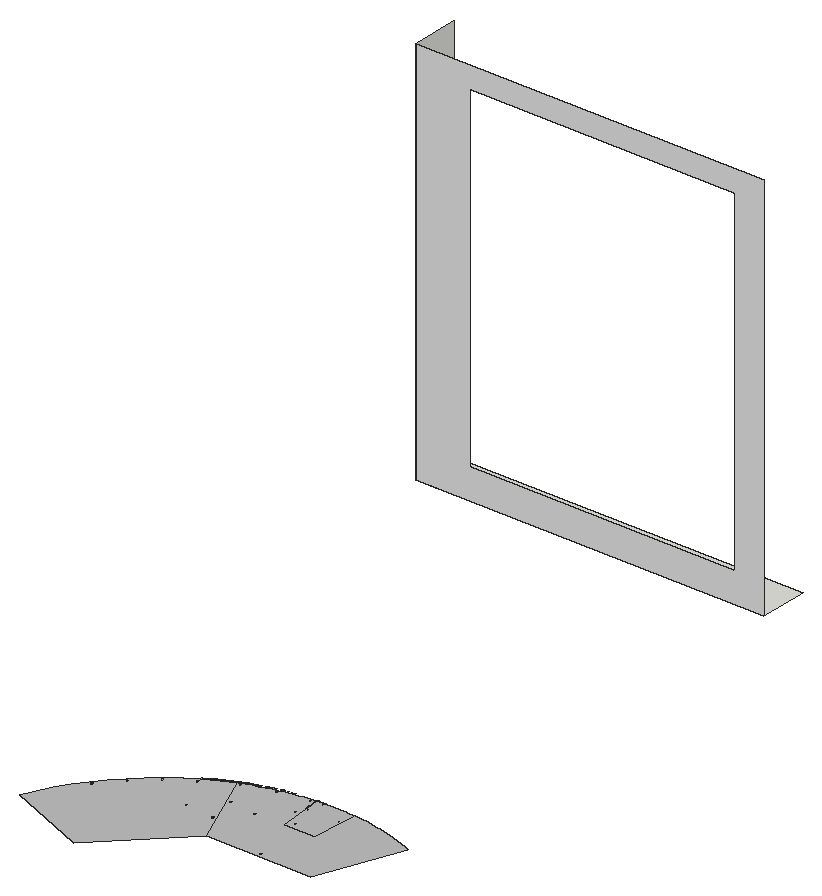
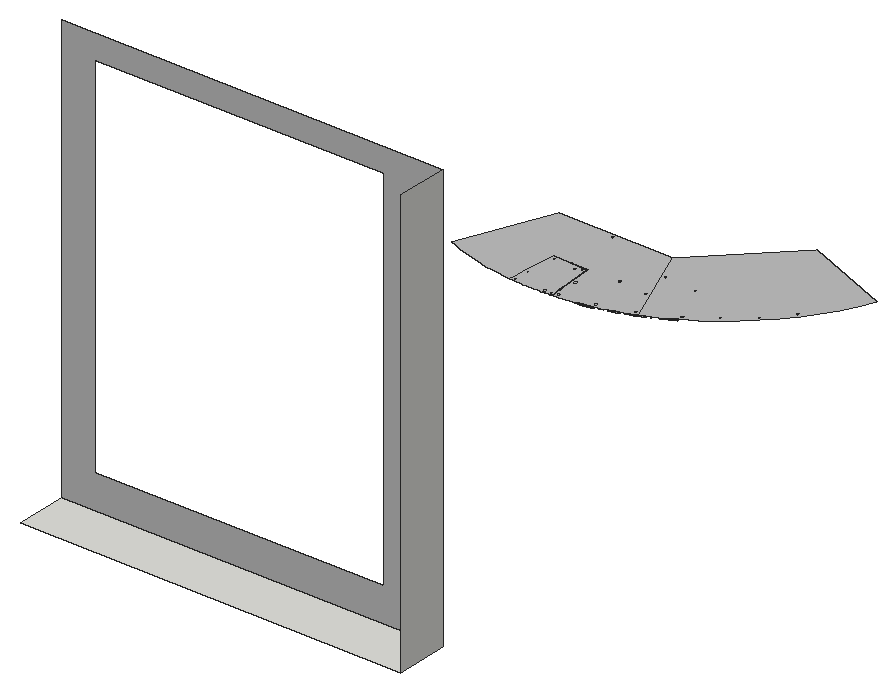
# SketchUp Ruby script. Lengths in inches.
U = 1.inch
M = Sketchup.active_model
def pt(a) = Geom::Point3d.new(a.map { |v| v * U })
def face(e, loops, mat)
  f = e.add_face(loops[0].map { |a| pt(a) })
  loops[1..].each { |l| e.add_face(l.map { |a| pt(a) }).erase! }
  f.material = f.back_material = mat if mat
  f
end
# faces: each face lists its corners as indices into pts; further lists are holes
def faces(e, pts, list, mat = nil) = list.each { |f| face(e, (f[0].is_a?(Array) ? f : [f]).map { |l| l.map { |i| pts[i] } }, mat) }
# xy, xz, yz: faces in a plane at the given z, y or x. An outline is a flat list of corners, or four numbers for a rectangle; further outlines are holes
def ring(l) = l.size == 4 ? [[l[0], l[1]], [l[2], l[1]], [l[2], l[3]], [l[0], l[3]]] : l.each_slice(2).to_a
def flat(e, list, mat, &to3) = list.each { |f| face(e, (f[0].is_a?(Array) ? f : [f]).map { |l| ring(l).map { |u, v| to3.(u, v) } }, mat) }
def xy(e, z, list, mat = nil) = flat(e, list, mat) { |x, y| [x, y, z] }
def xz(e, y, list, mat = nil) = flat(e, list, mat) { |x, z| [x, y, z] }
def yz(e, x, list, mat = nil) = flat(e, list, mat) { |y, z| [x, y, z] }
def lines(e, pts, list) = list.each { |a, b| e.add_line(pt(pts[a]), pt(pts[b])) }
# prism: a flat outline (further loops are holes) pulled along v
def prism(e, loops, v, mat = nil)
  f = face(e, loops, mat); d = Geom::Vector3d.new(v.map { |x| x * U })
  f.pushpull(f.normal.samedirection?(d) ? d.length : -d.length)
end
def box(e, o, s, mat = nil) = prism(e, [[o, [o[0] + s[0], o[1], o[2]], [o[0] + s[0], o[1] + s[1], o[2]], [o[0], o[1] + s[1], o[2]]]], [0, 0, s[2]], mat)
def at(x, y, z, deg = 0) = Geom::Transformation.translation(pt([x, y, z])) * Geom::Transformation.rotation(ORIGIN, Z_AXIS, deg.degrees)
def axes(o, x, y, z) = Geom::Transformation.new([*x, 0, *y, 0, *z, 0, *pt(o).to_a, 1])
def part(name) = M.definitions.add(name)
# library, detail: a bought-in or finely detailed component or shape, given as its bounding box
def library(name, o, s) = part(name).tap { |d| box(d.entities, o, s) }
def detail(e, o, s) = box(e.add_group.entities, o, s)
def put(e, d, t, mat = nil) = e.add_instance(d, t).tap { |i| i.material = mat if mat }
def group(e, t, mat = nil) = e.add_group.tap { |g| g.transformation = t; g.material = mat if mat }.entities
root = M.entities
M.materials.add("[Metal_Steel_Textured_White]").color = [191, 191, 191]
M.materials.add("[Polished Concrete Old]").color = [229, 229, 229]
xy(root,3.625,[[116.615,243.402,158.149,249.09]])
xy(root,3.625,[[[134.847,169.578,125.229,173.5625,125.948,175.149,126.769,176.685,127.689,178.164,128.703,179.579,129.808,180.926,130.999,182.197,132.27,183.387,133.616,184.492,135.032,185.507,136.511,186.426,138.047,187.247,139.633,187.966,143.617,178.348],[141.048,176.255,141.071,176.258,141.092,176.267,141.111,176.281,141.125,176.299,141.134,176.321,141.137,176.344,141.134,176.367,141.125,176.388,141.111,176.407,141.092,176.421,141.071,176.43,141.048,176.433,141.025,176.43,141.003,176.421,140.985,176.407,140.971,176.388,140.962,176.367,140.959,176.344,140.962,176.321,140.971,176.299,140.985,176.281,141.003,176.267,141.025,176.258],[138.462,181.667,138.485,181.67,138.507,181.679,138.525,181.693,138.539,181.712,138.548,181.733,138.551,181.756,138.548,181.779,138.539,181.801,138.525,181.819,138.507,181.833,138.485,181.842,138.462,181.845,138.439,181.842,138.418,181.833,138.399,181.819,138.385,181.801,138.376,181.779,138.373,181.756,138.376,181.733,138.385,181.712,138.399,181.693,138.418,181.679,138.439,181.67],[125.754,173.688,125.777,173.691,125.798,173.7,125.817,173.714,125.831,173.733,125.84,173.754,125.843,173.777,125.84,173.8,125.831,173.822,125.817,173.84,125.798,173.854,125.777,173.863,125.754,173.866,125.731,173.863,125.709,173.854,125.691,173.84,125.677,173.822,125.668,173.8,125.665,173.777,125.668,173.754,125.677,173.733,125.691,173.714,125.709,173.7,125.731,173.691],[128.754,172.446,128.777,172.449,128.798,172.458,128.816,172.472,128.831,172.49,128.839,172.512,128.843,172.535,128.839,172.558,128.831,172.579,128.816,172.597,128.798,172.612,128.777,172.62,128.754,172.624,128.731,172.62,128.709,172.612,128.691,172.597,128.677,172.579,128.668,172.558,128.665,172.535,128.668,172.512,128.677,172.49,128.691,172.472,128.709,172.458,128.731,172.449],[143.146,178.353,143.169,178.356,143.19,178.365,143.209,178.379,143.223,178.397,143.232,178.419,143.235,178.442,143.232,178.465,143.223,178.486,143.209,178.505,143.19,178.519,143.169,178.528,143.146,178.531,143.123,178.528,143.101,178.519,143.083,178.505,143.069,178.486,143.06,178.465,143.057,178.442,143.06,178.419,143.069,178.397,143.083,178.379,143.101,178.365,143.123,178.356],[134.754,169.961,134.777,169.964,134.798,169.972,134.816,169.987,134.831,170.005,134.839,170.026,134.842,170.049,134.839,170.072,134.831,170.094,134.816,170.112,134.798,170.126,134.777,170.135,134.754,170.138,134.731,170.135,134.709,170.126,134.691,170.112,134.677,170.094,134.668,170.072,134.665,170.049,134.668,170.026,134.677,170.005,134.691,169.987,134.709,169.972,134.731,169.964],[140.661,184.353,140.684,184.356,140.705,184.365,140.724,184.379,140.738,184.397,140.747,184.419,140.75,184.442,140.747,184.465,140.738,184.486,140.724,184.505,140.705,184.519,140.684,184.528,140.661,184.531,140.638,184.528,140.616,184.519,140.598,184.505,140.584,184.486,140.575,184.465,140.572,184.442,140.575,184.419,140.584,184.397,140.598,184.379,140.616,184.365,140.638,184.356],[136.48,185.857,136.503,185.86,136.525,185.869,136.543,185.883,136.557,185.902,136.566,185.923,136.569,185.946,136.566,185.969,136.557,185.991,136.543,186.009,136.525,186.023,136.503,186.032,136.48,186.035,136.457,186.032,136.436,186.023,136.418,186.009,136.403,185.991,136.395,185.969,136.392,185.946,136.395,185.923,136.403,185.902,136.418,185.883,136.436,185.869,136.457,185.86],[131.754,171.203,131.777,171.206,131.798,171.215,131.816,171.229,131.831,171.248,131.839,171.269,131.842,171.292,131.839,171.315,131.831,171.336,131.816,171.355,131.798,171.369,131.777,171.378,131.754,171.381,131.731,171.378,131.709,171.369,131.691,171.355,131.677,171.336,131.668,171.315,131.665,171.292,131.668,171.269,131.677,171.248,131.691,171.229,131.709,171.215,131.731,171.206],[131.439,174.644,131.462,174.647,131.483,174.656,131.502,174.67,131.516,174.689,131.525,174.71,131.528,174.733,131.525,174.756,131.516,174.778,131.502,174.796,131.483,174.81,131.462,174.819,131.439,174.822,131.416,174.819,131.395,174.81,131.376,174.796,131.362,174.778,131.353,174.756,131.35,174.733,131.353,174.71,131.362,174.689,131.376,174.67,131.395,174.656,131.416,174.647],[138.95,174.157,138.973,174.16,138.994,174.169,139.013,174.183,139.027,174.201,139.036,174.223,139.039,174.246,139.036,174.269,139.027,174.29,139.013,174.308,138.994,174.323,138.973,174.331,138.95,174.334,138.927,174.331,138.905,174.323,138.887,174.308,138.873,174.29,138.864,174.269,138.861,174.246,138.864,174.223,138.873,174.201,138.887,174.183,138.905,174.169,138.927,174.16],[127.249,176.626,127.272,176.629,127.293,176.638,127.312,176.652,127.326,176.67,127.335,176.692,127.338,176.715,127.335,176.738,127.326,176.759,127.312,176.778,127.293,176.792,127.272,176.801,127.249,176.804,127.226,176.801,127.205,176.792,127.186,176.778,127.172,176.759,127.163,176.738,127.16,176.715,127.163,176.692,127.172,176.67,127.186,176.652,127.205,176.638,127.226,176.629],[133.754,184.005,133.777,184.008,133.798,184.017,133.816,184.031,133.831,184.05,133.839,184.071,133.843,184.094,133.839,184.117,133.831,184.139,133.816,184.157,133.798,184.171,133.777,184.18,133.754,184.183,133.731,184.18,133.709,184.171,133.691,184.157,133.677,184.139,133.668,184.117,133.665,184.094,133.668,184.071,133.677,184.05,133.691,184.031,133.709,184.017,133.731,184.008],[129.101,179.353,129.124,179.356,129.146,179.365,129.164,179.379,129.178,179.397,129.187,179.419,129.19,179.442,129.187,179.465,129.178,179.486,129.164,179.505,129.146,179.519,129.124,179.528,129.101,179.531,129.078,179.528,129.057,179.519,129.038,179.505,129.024,179.486,129.015,179.465,129.012,179.442,129.015,179.419,129.024,179.397,129.038,179.379,129.057,179.365,129.078,179.356],[133.78,176.985,133.803,176.988,133.825,176.997,133.843,177.011,133.857,177.03,133.866,177.051,133.869,177.074,133.866,177.097,133.857,177.119,133.843,177.137,133.825,177.151,133.803,177.16,133.78,177.163,133.757,177.16,133.736,177.151,133.717,177.137,133.703,177.119,133.694,177.097,133.691,177.074,133.694,177.051,133.703,177.03,133.717,177.011,133.736,176.997,133.757,176.988],[136.852,172.059,136.875,172.062,136.896,172.071,136.914,172.085,136.929,172.103,136.9375,172.124,136.941,172.147,136.9375,172.17,136.929,172.192,136.914,172.21,136.896,172.224,136.875,172.233,136.852,172.236,136.829,172.233,136.807,172.224,136.789,172.21,136.775,172.192,136.766,172.17,136.763,172.147,136.766,172.124,136.775,172.103,136.789,172.085,136.807,172.071,136.829,172.062],[131.281,181.826,131.304,181.829,131.325,181.837,131.344,181.852,131.358,181.87,131.367,181.891,131.37,181.914,131.367,181.9375,131.358,181.959,131.344,181.977,131.325,181.991,131.304,182,131.281,182.003,131.258,182,131.236,181.991,131.218,181.977,131.204,181.959,131.195,181.9375,131.192,181.914,131.195,181.891,131.204,181.87,131.218,181.852,131.236,181.837,131.258,181.829],[136.121,179.326,136.144,179.329,136.166,179.338,136.184,179.352,136.198,179.371,136.207,179.392,136.21,179.415,136.207,179.438,136.198,179.46,136.184,179.478,136.166,179.492,136.144,179.501,136.121,179.504,136.098,179.501,136.077,179.492,136.058,179.478,136.044,179.46,136.035,179.438,136.032,179.415,136.035,179.392,136.044,179.371,136.058,179.352,136.077,179.338,136.098,179.329],[139.418,187.353,139.441,187.356,139.462,187.365,139.481,187.379,139.495,187.397,139.504,187.419,139.507,187.442,139.504,187.465,139.495,187.486,139.481,187.505,139.462,187.519,139.441,187.528,139.418,187.531,139.395,187.528,139.374,187.519,139.355,187.505,139.341,187.486,139.332,187.465,139.329,187.442,139.332,187.419,139.341,187.397,139.355,187.379,139.374,187.365,139.395,187.356],[141.903,181.353,141.926,181.356,141.948,181.365,141.966,181.379,141.98,181.397,141.989,181.419,141.992,181.442,141.989,181.465,141.98,181.486,141.966,181.505,141.948,181.519,141.926,181.528,141.903,181.531,141.88,181.528,141.859,181.519,141.84,181.505,141.826,181.486,141.817,181.465,141.814,181.442,141.817,181.419,141.826,181.397,141.84,181.379,141.859,181.365,141.88,181.356]],[[143.617,178.348,139.633,187.966,140.262,188.217,140.897,188.452,141.538,188.671,142.185,188.874,142.836,189.06,143.492,189.229,144.152,189.382,144.816,189.518,145.483,189.636,146.152,189.738,146.824,189.823,147.498,189.891,147.513,189.727,147.542,189.396,147.548,189.326,147.59,188.846,147.62,188.494,147.627,188.414,147.634,188.34,147.643,188.234,147.655,188.101,147.97,184.503,151.666,184.503,151.981,188.101,151.993,188.234,152.002,188.34,152.094,189.396,152.123,189.727,152.138,189.891,152.812,189.823,153.484,189.738,154.153,189.636,154.82,189.518,155.484,189.382,156.144,189.229,156.8,189.06,157.451,188.874,158.097,188.671,158.738,188.452,159.374,188.217,160.003,187.966,156.019,178.348],[147.136,189.366,147.159,189.369,147.18,189.378,147.198,189.392,147.213,189.411,147.222,189.432,147.225,189.455,147.222,189.478,147.213,189.5,147.198,189.518,147.18,189.532,147.159,189.541,147.136,189.544,147.113,189.541,147.091,189.532,147.073,189.518,147.059,189.5,147.05,189.478,147.047,189.455,147.05,189.432,147.059,189.411,147.073,189.392,147.091,189.378,147.113,189.369],[152.5,189.366,152.523,189.369,152.545,189.378,152.563,189.392,152.577,189.411,152.586,189.432,152.589,189.455,152.586,189.478,152.577,189.5,152.563,189.518,152.545,189.532,152.523,189.541,152.5,189.544,152.477,189.541,152.456,189.532,152.437,189.518,152.423,189.5,152.414,189.478,152.411,189.455,152.414,189.432,152.423,189.411,152.437,189.392,152.456,189.378,152.477,189.369],[142.641,181.658,142.664,181.661,142.685,181.67,142.704,181.684,142.718,181.703,142.727,181.724,142.73,181.747,142.727,181.77,142.718,181.792,142.704,181.81,142.685,181.824,142.664,181.833,142.641,181.836,142.618,181.833,142.597,181.824,142.578,181.81,142.564,181.792,142.555,181.77,142.552,181.747,142.555,181.724,142.564,181.703,142.578,181.684,142.597,181.67,142.618,181.661],[159.48,187.658,159.503,187.661,159.525,187.67,159.543,187.684,159.557,187.703,159.566,187.724,159.569,187.747,159.566,187.77,159.557,187.792,159.543,187.81,159.525,187.824,159.503,187.833,159.48,187.836,159.457,187.833,159.436,187.824,159.417,187.81,159.403,187.792,159.394,187.77,159.391,187.747,159.394,187.724,159.403,187.703,159.417,187.684,159.436,187.67,159.457,187.661],[156.995,181.658,157.018,181.661,157.039,181.67,157.058,181.684,157.072,181.703,157.081,181.724,157.084,181.747,157.081,181.77,157.072,181.792,157.058,181.81,157.039,181.824,157.018,181.833,156.995,181.836,156.972,181.833,156.95,181.824,156.932,181.81,156.918,181.792,156.909,181.77,156.906,181.747,156.909,181.724,156.918,181.703,156.932,181.684,156.95,181.67,156.972,181.661],[141.398,184.658,141.421,184.661,141.443,184.67,141.461,184.684,141.475,184.703,141.484,184.724,141.487,184.747,141.484,184.77,141.475,184.792,141.461,184.81,141.443,184.824,141.421,184.833,141.398,184.836,141.375,184.833,141.354,184.824,141.335,184.81,141.321,184.792,141.3125,184.77,141.309,184.747,141.3125,184.724,141.321,184.703,141.335,184.684,141.354,184.67,141.375,184.661],[158.237,184.658,158.26,184.661,158.282,184.67,158.3,184.684,158.314,184.703,158.323,184.724,158.326,184.747,158.323,184.77,158.314,184.792,158.3,184.81,158.282,184.824,158.26,184.833,158.237,184.836,158.214,184.833,158.193,184.824,158.175,184.81,158.16,184.792,158.152,184.77,158.149,184.747,158.152,184.724,158.16,184.703,158.175,184.684,158.193,184.67,158.214,184.661],[140.156,187.658,140.179,187.661,140.2,187.67,140.219,187.684,140.233,187.703,140.242,187.724,140.245,187.747,140.242,187.77,140.233,187.792,140.219,187.81,140.2,187.824,140.179,187.833,140.156,187.836,140.133,187.833,140.111,187.824,140.093,187.81,140.079,187.792,140.07,187.77,140.067,187.747,140.07,187.724,140.079,187.703,140.093,187.684,140.111,187.67,140.133,187.661],[156.049,188.753,156.072,188.756,156.093,188.764,156.112,188.779,156.126,188.797,156.135,188.818,156.138,188.841,156.135,188.864,156.126,188.886,156.112,188.904,156.093,188.918,156.072,188.927,156.049,188.93,156.026,188.927,156.004,188.918,155.986,188.904,155.972,188.886,155.963,188.864,155.96,188.841,155.963,188.818,155.972,188.797,155.986,188.779,156.004,188.764,156.026,188.756],[143.884,178.658,143.907,178.661,143.928,178.67,143.946,178.684,143.961,178.703,143.969,178.724,143.972,178.747,143.969,178.77,143.961,178.792,143.946,178.81,143.928,178.824,143.907,178.833,143.884,178.836,143.861,178.833,143.839,178.824,143.821,178.81,143.807,178.792,143.798,178.77,143.795,178.747,143.798,178.724,143.807,178.703,143.821,178.684,143.839,178.67,143.861,178.661],[143.587,188.753,143.61,188.756,143.631,188.764,143.65,188.779,143.664,188.797,143.673,188.818,143.676,188.841,143.673,188.864,143.664,188.886,143.65,188.904,143.631,188.918,143.61,188.927,143.587,188.93,143.564,188.927,143.542,188.918,143.524,188.904,143.51,188.886,143.501,188.864,143.498,188.841,143.501,188.818,143.51,188.797,143.524,188.779,143.542,188.764,143.564,188.756],[144.559,184.314,144.582,184.317,144.604,184.326,144.622,184.34,144.636,184.358,144.645,184.38,144.648,184.403,144.645,184.426,144.636,184.447,144.622,184.466,144.604,184.48,144.582,184.489,144.559,184.492,144.536,184.489,144.515,184.48,144.496,184.466,144.482,184.447,144.473,184.426,144.47,184.403,144.473,184.38,144.482,184.358,144.496,184.34,144.515,184.326,144.536,184.317],[155.076,184.314,155.099,184.317,155.121,184.326,155.139,184.34,155.153,184.358,155.162,184.38,155.165,184.403,155.162,184.426,155.153,184.447,155.139,184.466,155.121,184.48,155.099,184.489,155.076,184.492,155.053,184.489,155.032,184.48,155.014,184.466,154.999,184.447,154.991,184.426,154.988,184.403,154.991,184.38,154.999,184.358,155.014,184.34,155.032,184.326,155.053,184.317],[152.058,184.314,152.081,184.317,152.103,184.326,152.121,184.34,152.135,184.358,152.144,184.38,152.147,184.403,152.144,184.426,152.135,184.447,152.121,184.466,152.103,184.48,152.081,184.489,152.058,184.492,152.035,184.489,152.014,184.48,151.995,184.466,151.981,184.447,151.972,184.426,151.969,184.403,151.972,184.38,151.981,184.358,151.995,184.34,152.014,184.326,152.035,184.317],[147.578,184.314,147.601,184.317,147.622,184.326,147.641,184.34,147.655,184.358,147.664,184.38,147.667,184.403,147.664,184.426,147.655,184.447,147.641,184.466,147.622,184.48,147.601,184.489,147.578,184.492,147.555,184.489,147.533,184.48,147.515,184.466,147.501,184.447,147.492,184.426,147.489,184.403,147.492,184.38,147.501,184.358,147.515,184.34,147.533,184.326,147.555,184.317],[147.357,186.84,147.38,186.843,147.401,186.852,147.42,186.866,147.434,186.885,147.443,186.906,147.446,186.929,147.443,186.952,147.434,186.973,147.42,186.992,147.401,187.006,147.38,187.015,147.357,187.018,147.334,187.015,147.312,187.006,147.294,186.992,147.28,186.973,147.271,186.952,147.268,186.929,147.271,186.906,147.28,186.885,147.294,186.866,147.312,186.852,147.334,186.843],[152.279,186.84,152.302,186.843,152.324,186.852,152.342,186.866,152.356,186.885,152.365,186.906,152.368,186.929,152.365,186.952,152.356,186.973,152.342,186.992,152.324,187.006,152.302,187.015,152.279,187.018,152.256,187.015,152.235,187.006,152.216,186.992,152.202,186.973,152.193,186.952,152.19,186.929,152.193,186.906,152.202,186.885,152.216,186.866,152.235,186.852,152.256,186.843],[155.752,178.658,155.775,178.661,155.797,178.67,155.815,178.684,155.829,178.703,155.838,178.724,155.841,178.747,155.838,178.77,155.829,178.792,155.815,178.81,155.797,178.824,155.775,178.833,155.752,178.836,155.729,178.833,155.708,178.824,155.689,178.81,155.675,178.792,155.666,178.77,155.663,178.747,155.666,178.724,155.675,178.703,155.689,178.684,155.708,178.67,155.729,178.661],[146.851,178.658,146.874,178.661,146.895,178.67,146.914,178.684,146.928,178.703,146.937,178.724,146.94,178.747,146.937,178.77,146.928,178.792,146.914,178.81,146.895,178.824,146.874,178.833,146.851,178.836,146.828,178.833,146.806,178.824,146.788,178.81,146.774,178.792,146.765,178.77,146.762,178.747,146.765,178.724,146.774,178.703,146.788,178.684,146.806,178.67,146.828,178.661],[149.818,178.658,149.841,178.661,149.862,178.67,149.881,178.684,149.895,178.703,149.904,178.724,149.907,178.747,149.904,178.77,149.895,178.792,149.881,178.81,149.862,178.824,149.841,178.833,149.818,178.836,149.795,178.833,149.773,178.824,149.755,178.81,149.741,178.792,149.732,178.77,149.729,178.747,149.732,178.724,149.741,178.703,149.755,178.684,149.773,178.67,149.795,178.661],[152.785,178.658,152.808,178.661,152.829,178.67,152.848,178.684,152.862,178.703,152.871,178.724,152.874,178.747,152.871,178.77,152.862,178.792,152.848,178.81,152.829,178.824,152.808,178.833,152.785,178.836,152.762,178.833,152.741,178.824,152.722,178.81,152.708,178.792,152.699,178.77,152.696,178.747,152.699,178.724,152.708,178.703,152.722,178.684,152.741,178.67,152.762,178.661]],[149.818,178.659,149.795,178.662,149.774,178.671,149.756,178.685,149.742,178.703,149.733,178.725,149.73,178.747,149.733,178.77,149.742,178.791,149.756,178.809,149.774,178.823,149.795,178.832,149.818,178.835,149.818,178.784,149.808,178.783,149.8,178.779,149.792,178.773,149.786,178.766,149.783,178.757,149.781,178.747,149.783,178.738,149.786,178.729,149.792,178.721,149.8,178.716,149.808,178.712,149.818,178.711],[149.818,178.727,149.813,178.728,149.808,178.73,149.804,178.733,149.801,178.737,149.799,178.742,149.798,178.747,149.799,178.752,149.801,178.757,149.804,178.761,149.808,178.765,149.813,178.767,149.818,178.767],[[129.101,179.353,129.078,179.356,129.057,179.365,129.038,179.379,129.024,179.397,129.015,179.419,129.012,179.442,129.015,179.465,129.024,179.486,129.038,179.505,129.057,179.519,129.078,179.528,129.101,179.531,129.124,179.528,129.146,179.519,129.164,179.505,129.178,179.486,129.187,179.465,129.19,179.442,129.187,179.419,129.178,179.397,129.164,179.379,129.146,179.365,129.124,179.356],[129.101,179.354,129.124,179.357,129.145,179.366,129.163,179.38,129.177,179.398,129.186,179.419,129.189,179.442,129.186,179.464,129.177,179.486,129.163,179.504,129.145,179.518,129.124,179.527,129.101,179.53,129.078,179.527,129.057,179.518,129.039,179.504,129.025,179.486,129.016,179.464,129.013,179.442,129.016,179.419,129.025,179.398,129.039,179.38,129.057,179.366,129.078,179.357]],
  [[129.101,179.405,129.092,179.406,129.083,179.41,129.075,179.416,129.069,179.423,129.066,179.432,129.065,179.442,129.066,179.451,129.069,179.46,129.075,179.468,129.083,179.473,129.092,179.477,129.101,179.478,129.111,179.477,129.119,179.473,129.127,179.468,129.133,179.46,129.137,179.451,129.138,179.442,129.137,179.432,129.133,179.423,129.127,179.416,129.119,179.41,129.111,179.406],[129.096,179.422,129.106,179.422,129.111,179.424,129.115,179.428,129.118,179.432,129.12,179.437,129.121,179.442,129.12,179.447,129.118,179.452,129.115,179.456,129.111,179.459,129.106,179.461,129.101,179.462,129.096,179.461,129.091,179.459,129.087,179.456,129.084,179.452,129.082,179.447,129.081,179.442,129.082,179.437,129.084,179.432,129.087,179.428,129.091,179.424]],[129.096,179.422,129.091,179.424,129.087,179.428,129.084,179.432,129.082,179.437,129.081,179.442,129.082,179.447,129.084,179.452,129.087,179.456,129.091,179.459,129.096,179.461,129.101,179.462,129.106,179.461,129.111,179.459,129.115,179.456,129.118,179.452,129.12,179.447,129.121,179.442,129.12,179.437,129.118,179.432,129.115,179.428,129.111,179.424,129.106,179.422],[[141.903,181.354,141.881,181.357,141.859,181.366,141.841,181.38,141.827,181.398,141.818,181.419,141.815,181.442,141.818,181.464,141.827,181.486,141.841,181.504,141.859,181.518,141.881,181.527,141.903,181.53,141.926,181.527,141.947,181.518,141.965,181.504,141.979,181.486,141.988,181.464,141.991,181.442,141.988,181.419,141.979,181.398,141.965,181.38,141.947,181.366,141.926,181.357],[141.903,181.405,141.913,181.406,141.922,181.41,141.929,181.416,141.935,181.423,141.939,181.432,141.94,181.442,141.939,181.451,141.935,181.46,141.929,181.468,141.922,181.473,141.913,181.477,141.903,181.478,141.894,181.477,141.885,181.473,141.877,181.468,141.872,181.46,141.868,181.451,141.867,181.442,141.868,181.432,141.872,181.423,141.877,181.416,141.885,181.41,141.894,181.406]],[[141.903,181.405,141.894,181.406,141.885,181.41,141.877,181.416,141.872,181.423,141.868,181.432,141.867,181.442,141.868,181.451,141.872,181.46,141.877,181.468,141.885,181.473,141.894,181.477,141.903,181.478,141.913,181.477,141.922,181.473,141.929,181.468,141.935,181.46,141.939,181.451,141.94,181.442,141.939,181.432,141.935,181.423,141.929,181.416,141.922,181.41,141.913,181.406],[141.898,181.422,141.908,181.422,141.913,181.424,141.921,181.432,141.923,181.437,141.923,181.447,141.921,181.452,141.917,181.456,141.913,181.459,141.908,181.461,141.903,181.462,141.898,181.461,141.893,181.459,141.889,181.456,141.886,181.452,141.884,181.447,141.883,181.442,141.884,181.437,141.886,181.432,141.889,181.428,141.893,181.424]],[141.898,181.422,141.893,181.424,141.889,181.428,141.886,181.432,141.884,181.437,141.883,181.442,141.884,181.447,141.886,181.452,141.889,181.456,141.893,181.459,141.898,181.461,141.903,181.462,141.908,181.461,141.913,181.459,141.917,181.456,141.921,181.452,141.923,181.447,141.923,181.437,141.921,181.432,141.913,181.424,141.908,181.422],
  [[138.462,181.72,138.453,181.721,138.444,181.725,138.436,181.73,138.431,181.738,138.427,181.747,138.426,181.756,138.427,181.766,138.431,181.775,138.436,181.782,138.444,181.788,138.453,181.792,138.462,181.793,138.472,181.792,138.481,181.788,138.488,181.782,138.494,181.775,138.498,181.766,138.499,181.756,138.498,181.747,138.494,181.738,138.488,181.73,138.481,181.725,138.472,181.721],[138.462,181.736,138.467,181.737,138.472,181.739,138.476,181.742,138.48,181.746,138.482,181.751,138.482,181.761,138.48,181.766,138.472,181.774,138.467,181.776,138.457,181.776,138.452,181.774,138.448,181.77,138.445,181.766,138.443,181.761,138.442,181.756,138.443,181.751,138.445,181.746,138.448,181.742,138.452,181.739,138.457,181.737]],[138.462,181.736,138.457,181.737,138.452,181.739,138.448,181.742,138.445,181.746,138.443,181.751,138.442,181.756,138.443,181.761,138.445,181.766,138.448,181.77,138.452,181.774,138.457,181.776,138.467,181.776,138.472,181.774,138.48,181.766,138.482,181.761,138.482,181.751,138.48,181.746,138.476,181.742,138.472,181.739,138.467,181.737],[[131.281,181.878,131.271,181.879,131.263,181.883,131.255,181.889,131.249,181.896,131.246,181.905,131.244,181.914,131.246,181.924,131.249,181.933,131.255,181.94,131.263,181.946,131.271,181.95,131.281,181.951,131.29,181.95,131.299,181.946,131.307,181.94,131.3125,181.933,131.316,181.924,131.317,181.914,131.316,181.905,131.3125,181.896,131.307,181.889,131.299,181.883,131.29,181.879],[131.281,181.894,131.286,181.895,131.291,181.897,131.295,181.9,131.298,181.904,131.3,181.909,131.301,181.914,131.3,181.92,131.298,181.924,131.295,181.929,131.291,181.932,131.286,181.934,131.276,181.934,131.271,181.932,131.267,181.929,131.264,181.924,131.262,181.92,131.261,181.914,131.262,181.909,131.264,181.904,131.267,181.9,131.271,181.897,131.276,181.895]],[131.281,181.894,131.276,181.895,131.271,181.897,131.267,181.9,131.264,181.904,131.262,181.909,131.261,181.914,131.262,181.92,131.264,181.924,131.267,181.929,131.271,181.932,131.276,181.934,131.286,181.934,131.291,181.932,131.295,181.929,131.298,181.924,131.3,181.92,131.301,181.914,131.3,181.909,131.298,181.904,131.295,181.9,131.291,181.897,131.286,181.895],[[133.754,184.006,133.731,184.009,133.71,184.018,133.691,184.032,133.677,184.05,133.669,184.071,133.666,184.094,133.669,184.117,133.677,184.138,133.691,184.156,133.71,184.17,133.731,184.179,133.754,184.182,133.776,184.179,133.798,184.17,133.816,184.156,133.83,184.138,133.839,184.117,133.842,184.094,133.839,184.071,133.83,184.05,133.816,184.032,133.798,184.018,133.776,184.009],[133.754,184.058,133.763,184.059,133.772,184.0625,133.78,184.068,133.785,184.076,133.789,184.085,133.79,184.094,133.789,184.104,133.785,184.112,133.78,184.12,133.772,184.126,133.763,184.13,133.754,184.131,133.744,184.13,133.735,184.126,133.728,184.12,133.722,184.112,133.718,184.104,133.717,184.094,133.718,184.085,133.722,184.076,133.728,184.068,133.735,184.0625,133.744,184.059]],
  [[144.559,184.314,144.536,184.317,144.515,184.326,144.496,184.34,144.482,184.358,144.473,184.38,144.47,184.403,144.473,184.426,144.482,184.447,144.496,184.466,144.515,184.48,144.536,184.489,144.559,184.492,144.582,184.489,144.604,184.48,144.622,184.466,144.636,184.447,144.645,184.426,144.648,184.403,144.645,184.38,144.636,184.358,144.622,184.34,144.604,184.326,144.582,184.317],[144.559,184.315,144.582,184.318,144.603,184.327,144.621,184.341,144.635,184.359,144.644,184.38,144.647,184.403,144.644,184.426,144.635,184.447,144.621,184.465,144.603,184.479,144.582,184.488,144.559,184.491,144.537,184.488,144.515,184.479,144.497,184.465,144.483,184.447,144.474,184.426,144.471,184.403,144.474,184.38,144.483,184.359,144.497,184.341,144.515,184.327,144.537,184.318]],[[144.559,184.366,144.55,184.368,144.541,184.371,144.533,184.377,144.528,184.385,144.524,184.393,144.523,184.403,144.524,184.412,144.528,184.421,144.533,184.429,144.541,184.435,144.55,184.438,144.559,184.44,144.569,184.438,144.578,184.435,144.585,184.429,144.591,184.421,144.595,184.412,144.596,184.403,144.595,184.393,144.591,184.385,144.585,184.377,144.578,184.371,144.569,184.368],[144.559,184.383,144.564,184.384,144.569,184.386,144.573,184.389,144.577,184.393,144.579,184.398,144.579,184.408,144.577,184.413,144.573,184.417,144.569,184.42,144.564,184.422,144.559,184.423,144.554,184.422,144.549,184.42,144.545,184.417,144.542,184.413,144.54,184.408,144.539,184.403,144.54,184.398,144.542,184.393,144.545,184.389,144.549,184.386,144.554,184.384]],[144.559,184.383,144.554,184.384,144.549,184.386,144.545,184.389,144.542,184.393,144.54,184.398,144.539,184.403,144.54,184.408,144.542,184.413,144.545,184.417,144.549,184.42,144.554,184.422,144.559,184.423,144.564,184.422,144.569,184.42,144.573,184.417,144.577,184.413,144.579,184.408,144.579,184.398,144.577,184.393,144.573,184.389,144.569,184.386,144.564,184.384],[147.97,184.503,147.655,188.101,147.663,188.111],[147.97,184.503,147.663,188.111,147.667,188.115,147.982,184.516,149.818,184.516,149.818,184.503],
  [[147.982,184.516,147.667,188.115,147.657,188.235,147.647,188.341,147.641,188.407,147.635,188.486,147.604,188.833,147.565,189.283,147.556,189.389,147.555,189.397,147.526,189.728,147.523,189.759,147.523,189.76,147.512,189.892,148.521,189.96,148.664,189.967,149.048,189.981,149.433,189.989,149.818,189.992,150.203,189.989,150.588,189.981,150.972,189.967,151.357,189.947,151.741,189.922,152.124,189.892,152.11,189.728,152.081,189.397,151.989,188.341,151.979,188.235,151.969,188.115,151.654,184.516],[151.361,184.669,151.404,184.675,151.444,184.691,151.479,184.718,151.505,184.752,151.522,184.792,151.528,184.835,151.522,184.878,151.505,184.919,151.479,184.953,151.444,184.979,151.404,184.996,151.361,185.002,151.318,184.996,151.278,184.979,151.244,184.953,151.217,184.919,151.201,184.878,151.195,184.835,151.201,184.792,151.217,184.752,151.244,184.718,151.278,184.691,151.318,184.675],[148.275,184.669,148.318,184.675,148.358,184.691,148.392,184.718,148.419,184.752,148.435,184.792,148.441,184.835,148.435,184.878,148.419,184.919,148.392,184.953,148.358,184.979,148.318,184.996,148.275,185.002,148.231,184.996,148.191,184.979,148.157,184.953,148.13,184.919,148.114,184.878,148.108,184.835,148.114,184.792,148.13,184.752,148.157,184.718,148.191,184.691,148.231,184.675],[151.644,187.895,151.687,187.901,151.727,187.917,151.761,187.944,151.788,187.978,151.804,188.018,151.81,188.062,151.804,188.105,151.788,188.145,151.761,188.179,151.727,188.206,151.687,188.222,151.644,188.228,151.6,188.222,151.56,188.206,151.526,188.179,151.499,188.145,151.483,188.105,151.477,188.062,151.483,188.018,151.499,187.978,151.526,187.944,151.56,187.917,151.6,187.901],[147.992,187.895,148.035,187.901,148.075,187.917,148.11,187.944,148.136,187.978,148.153,188.018,148.159,188.062,148.153,188.105,148.136,188.145,148.11,188.179,148.075,188.206,148.035,188.222,147.992,188.228,147.949,188.222,147.909,188.206,147.875,188.179,147.848,188.145,147.832,188.105,147.826,188.062,147.832,188.018,147.848,187.978,147.875,187.944,147.909,187.917,147.949,187.901],[147.859,189.42,147.902,189.426,147.942,189.442,147.976,189.469,148.003,189.503,148.02,189.543,148.025,189.586,148.02,189.629,148.003,189.669,147.976,189.704,147.942,189.73,147.902,189.747,147.859,189.753,147.816,189.747,147.776,189.73,147.741,189.704,147.715,189.669,147.698,189.629,147.693,189.586,147.698,189.543,147.715,189.503,147.741,189.469,147.776,189.442,147.816,189.426],[151.777,189.42,151.82,189.426,151.86,189.442,151.895,189.469,151.921,189.503,151.9375,189.543,151.943,189.586,151.9375,189.629,151.921,189.669,151.895,189.704,151.86,189.73,151.82,189.747,151.777,189.753,151.734,189.747,151.694,189.73,151.659,189.704,151.633,189.669,151.616,189.629,151.611,189.586,151.616,189.543,151.633,189.503,151.659,189.469,151.694,189.442,151.734,189.426],[151.094,189.473,151.117,189.476,151.138,189.485,151.156,189.499,151.17,189.517,151.179,189.539,151.182,189.562,151.179,189.585,151.17,189.606,151.156,189.625,151.138,189.639,151.117,189.648,151.094,189.651,151.07,189.648,151.049,189.639,151.031,189.625,151.017,189.606,151.008,189.585,151.005,189.562,151.008,189.539,151.017,189.517,151.031,189.499,151.049,189.485,151.07,189.476],[148.542,189.473,148.565,189.476,148.587,189.485,148.605,189.499,148.619,189.517,148.628,189.539,148.631,189.562,148.628,189.585,148.619,189.606,148.605,189.625,148.587,189.639,148.565,189.648,148.542,189.651,148.519,189.648,148.498,189.639,148.479,189.625,148.465,189.606,148.456,189.585,148.453,189.562,148.456,189.539,148.465,189.517,148.479,189.499,148.498,189.485,148.519,189.476],[148.82,185.093,148.843,185.096,148.864,185.104,148.883,185.119,148.897,185.137,148.906,185.158,148.909,185.181,148.906,185.204,148.897,185.226,148.883,185.244,148.864,185.258,148.843,185.267,148.82,185.27,148.797,185.267,148.775,185.258,148.757,185.244,148.743,185.226,148.734,185.204,148.731,185.181,148.734,185.158,148.743,185.137,148.757,185.119,148.775,185.104,148.797,185.096],[150.816,185.093,150.839,185.096,150.86,185.104,150.879,185.119,150.893,185.137,150.902,185.158,150.905,185.181,150.902,185.204,150.893,185.226,150.879,185.244,150.86,185.258,150.839,185.267,150.816,185.27,150.793,185.267,150.771,185.258,150.753,185.244,150.739,185.226,150.73,185.204,150.727,185.181,150.73,185.158,150.739,185.137,150.753,185.119,150.771,185.104,150.793,185.096],[149.818,185.128,149.832,185.13,149.845,185.135,149.856,185.144,149.864,185.155,149.869,185.168,149.871,185.181,149.869,185.195,149.864,185.208,149.856,185.219,149.845,185.227,149.832,185.233,149.818,185.235,149.804,185.233,149.791,185.227,149.78,185.219,149.772,185.208,149.766,185.195,149.765,185.181,149.766,185.168,149.772,185.155,149.78,185.144,149.791,185.135,149.804,185.13]],[[141.398,184.659,141.376,184.662,141.354,184.671,141.336,184.685,141.322,184.703,141.313,184.724,141.31,184.747,141.313,184.77,141.322,184.791,141.336,184.809,141.354,184.823,141.376,184.832,141.398,184.835,141.421,184.832,141.442,184.823,141.461,184.809,141.474,184.791,141.483,184.77,141.486,184.747,141.483,184.724,141.474,184.703,141.461,184.685,141.442,184.671,141.421,184.662],[141.398,184.711,141.408,184.712,141.417,184.716,141.424,184.721,141.43,184.729,141.434,184.738,141.435,184.747,141.434,184.757,141.43,184.766,141.424,184.773,141.417,184.779,141.408,184.783,141.398,184.784,141.389,184.783,141.38,184.779,141.372,184.773,141.367,184.766,141.363,184.757,141.362,184.747,141.363,184.738,141.367,184.729,141.372,184.721,141.38,184.716,141.389,184.712]],[[148.82,185.093,148.797,185.096,148.776,185.105,148.758,185.119,148.744,185.137,148.735,185.159,148.732,185.181,148.735,185.204,148.744,185.225,148.758,185.244,148.776,185.258,148.797,185.266,148.82,185.269,148.843,185.266,148.864,185.258,148.882,185.244,148.896,185.225,148.905,185.204,148.908,185.181,148.905,185.159,148.896,185.137,148.882,185.119,148.864,185.105,148.843,185.096],[148.82,185.145,148.829,185.146,148.838,185.15,148.846,185.156,148.852,185.163,148.855,185.172,148.856,185.181,148.855,185.191,148.852,185.2,148.846,185.207,148.838,185.213,148.829,185.217,148.82,185.218,148.81,185.217,148.802,185.213,148.794,185.207,148.788,185.2,148.784,185.191,148.783,185.181,148.784,185.172,148.788,185.163,148.794,185.156,148.802,185.15,148.81,185.146]],[[136.48,185.858,136.458,185.861,136.436,185.87,136.418,185.884,136.404,185.902,136.395,185.924,136.392,185.946,136.395,185.969,136.404,185.99,136.418,186.008,136.436,186.022,136.458,186.031,136.48,186.034,136.503,186.031,136.524,186.022,136.543,186.008,136.557,185.99,136.565,185.969,136.568,185.946,136.565,185.924,136.557,185.902,136.543,185.884,136.524,185.87,136.503,185.861],[136.48,185.91,136.49,185.911,136.499,185.915,136.506,185.92,136.512,185.928,136.516,185.937,136.517,185.946,136.516,185.956,136.512,185.965,136.506,185.972,136.499,185.978,136.49,185.982,136.48,185.983,136.471,185.982,136.462,185.978,136.455,185.972,136.449,185.965,136.445,185.956,136.444,185.946,136.445,185.937,136.449,185.928,136.455,185.92,136.462,185.915,136.471,185.911]],[[136.48,185.91,136.471,185.911,136.462,185.915,136.455,185.92,136.449,185.928,136.445,185.937,136.444,185.946,136.445,185.956,136.449,185.965,136.455,185.972,136.462,185.978,136.471,185.982,136.48,185.983,136.49,185.982,136.499,185.978,136.506,185.972,136.512,185.965,136.516,185.956,136.517,185.946,136.516,185.937,136.512,185.928,136.506,185.92,136.499,185.915,136.49,185.911],[136.48,185.926,136.486,185.927,136.49,185.929,136.495,185.932,136.498,185.936,136.5,185.941,136.5,185.951,136.498,185.956,136.495,185.96,136.49,185.964,136.486,185.966,136.475,185.966,136.47,185.964,136.466,185.96,136.463,185.956,136.461,185.951,136.46,185.946,136.461,185.941,136.463,185.936,136.466,185.932,136.47,185.929,136.475,185.927]],
  [136.48,185.926,136.475,185.927,136.47,185.929,136.466,185.932,136.463,185.936,136.461,185.941,136.46,185.946,136.461,185.951,136.463,185.956,136.466,185.96,136.47,185.964,136.475,185.966,136.486,185.966,136.49,185.964,136.495,185.96,136.498,185.956,136.5,185.951,136.5,185.941,136.498,185.936,136.495,185.932,136.49,185.929,136.486,185.927],[136.444,186.542,136.411,186.599,137.092,186.979,137.784,187.339,138.485,187.679,139.197,187.998,139.917,188.297,140.646,188.574,141.383,188.83,142.127,189.065,142.877,189.278,143.633,189.469,144.394,189.637,145.16,189.784,145.172,189.718,144.408,189.572,143.648,189.404,142.894,189.213,142.146,189.001,141.404,188.767,140.669,188.512,139.942,188.235,139.223,187.9375,138.514,187.619,137.813,187.28,137.123,186.921,136.454,186.547],[[147.357,186.841,147.334,186.844,147.3125,186.853,147.294,186.867,147.281,186.885,147.272,186.906,147.269,186.929,147.272,186.952,147.281,186.973,147.294,186.991,147.3125,187.005,147.334,187.014,147.357,187.017,147.379,187.014,147.401,187.005,147.419,186.991,147.433,186.973,147.442,186.952,147.445,186.929,147.442,186.906,147.433,186.885,147.419,186.867,147.401,186.853,147.379,186.844],[147.357,186.892,147.366,186.894,147.375,186.897,147.383,186.903,147.388,186.911,147.392,186.92,147.393,186.929,147.392,186.939,147.388,186.947,147.383,186.955,147.375,186.961,147.366,186.964,147.357,186.966,147.347,186.964,147.338,186.961,147.331,186.955,147.325,186.947,147.321,186.939,147.32,186.929,147.321,186.92,147.325,186.911,147.331,186.903,147.338,186.897,147.347,186.894]],[[140.156,187.658,140.133,187.661,140.111,187.67,140.093,187.684,140.079,187.703,140.07,187.724,140.067,187.747,140.07,187.77,140.079,187.792,140.093,187.81,140.111,187.824,140.133,187.833,140.156,187.836,140.179,187.833,140.2,187.824,140.219,187.81,140.233,187.792,140.242,187.77,140.245,187.747,140.242,187.724,140.233,187.703,140.219,187.684,140.2,187.67,140.179,187.661],[140.156,187.659,140.178,187.662,140.2,187.671,140.218,187.685,140.232,187.703,140.241,187.724,140.244,187.747,140.241,187.77,140.232,187.791,140.218,187.809,140.2,187.823,140.178,187.832,140.156,187.835,140.133,187.832,140.112,187.823,140.094,187.809,140.08,187.791,140.071,187.77,140.068,187.747,140.071,187.724,140.08,187.703,140.094,187.685,140.112,187.671,140.133,187.662]],[[140.156,187.659,140.133,187.662,140.112,187.671,140.094,187.685,140.08,187.703,140.071,187.724,140.068,187.747,140.071,187.77,140.08,187.791,140.094,187.809,140.112,187.823,140.133,187.832,140.156,187.835,140.178,187.832,140.2,187.823,140.218,187.809,140.232,187.791,140.241,187.77,140.244,187.747,140.241,187.724,140.232,187.703,140.218,187.685,140.2,187.671,140.178,187.662],[140.156,187.711,140.165,187.712,140.174,187.716,140.182,187.721,140.1875,187.729,140.191,187.738,140.192,187.747,140.191,187.757,140.1875,187.765,140.182,187.773,140.174,187.779,140.165,187.783,140.156,187.784,140.146,187.783,140.137,187.779,140.13,187.773,140.124,187.765,140.12,187.757,140.119,187.747,140.12,187.738,140.124,187.729,140.13,187.721,140.137,187.716,140.146,187.712]],
  [147.655,188.101,147.643,188.234,147.652,188.234,147.663,188.111],[147.663,188.111,147.652,188.234,147.657,188.235,147.667,188.115],[147.643,188.234,147.634,188.34,147.643,188.34,147.652,188.234],[147.652,188.234,147.643,188.34,147.647,188.341,147.657,188.235],[147.634,188.34,147.627,188.414,147.638,188.409,147.643,188.34],
  [147.643,188.34,147.638,188.409,147.641,188.407,147.647,188.341],[147.641,188.407,147.638,188.409,147.631,188.488,147.635,188.486],[147.638,188.409,147.627,188.414,147.62,188.494,147.626,188.491,147.631,188.488],[147.635,188.486,147.631,188.488,147.601,188.835,147.604,188.833],[147.631,188.488,147.626,188.491,147.62,188.494,147.59,188.846,147.601,188.835],
  [[143.587,188.753,143.564,188.756,143.542,188.764,143.524,188.779,143.51,188.797,143.501,188.818,143.498,188.841,143.501,188.864,143.51,188.886,143.524,188.904,143.542,188.918,143.564,188.927,143.587,188.93,143.61,188.927,143.631,188.918,143.65,188.904,143.664,188.886,143.673,188.864,143.676,188.841,143.673,188.818,143.664,188.797,143.65,188.779,143.631,188.764,143.61,188.756],[143.587,188.754,143.61,188.757,143.631,188.765,143.649,188.779,143.663,188.798,143.672,188.819,143.675,188.841,143.672,188.864,143.663,188.885,143.649,188.904,143.631,188.918,143.61,188.926,143.587,188.929,143.564,188.926,143.543,188.918,143.525,188.904,143.511,188.885,143.502,188.864,143.499,188.841,143.502,188.819,143.511,188.798,143.525,188.779,143.543,188.765,143.564,188.757]],[[143.587,188.805,143.577,188.806,143.569,188.81,143.561,188.816,143.555,188.823,143.552,188.832,143.55,188.841,143.552,188.851,143.555,188.86,143.561,188.867,143.569,188.873,143.577,188.877,143.587,188.878,143.596,188.877,143.605,188.873,143.613,188.867,143.619,188.86,143.622,188.851,143.623,188.841,143.622,188.832,143.619,188.823,143.613,188.816,143.605,188.81,143.596,188.806],[143.582,188.822,143.592,188.822,143.597,188.824,143.601,188.827,143.604,188.831,143.606,188.836,143.607,188.841,143.606,188.847,143.604,188.851,143.601,188.856,143.597,188.859,143.592,188.861,143.582,188.861,143.577,188.859,143.573,188.856,143.57,188.851,143.568,188.847,143.567,188.841,143.568,188.836,143.57,188.831,143.573,188.827,143.577,188.824]],[147.604,188.833,147.601,188.835,147.563,189.288,147.565,189.283],[147.601,188.835,147.59,188.846,147.548,189.326,147.56,189.294,147.563,189.288],[147.565,189.283,147.563,189.288,147.554,189.395,147.556,189.389],
  [147.563,189.288,147.56,189.294,147.548,189.326,147.542,189.396,147.554,189.397,147.554,189.395],[[147.136,189.366,147.113,189.369,147.091,189.378,147.073,189.392,147.059,189.411,147.05,189.432,147.047,189.455,147.05,189.478,147.059,189.5,147.073,189.518,147.091,189.532,147.113,189.541,147.136,189.544,147.159,189.541,147.18,189.532,147.198,189.518,147.213,189.5,147.222,189.478,147.225,189.455,147.222,189.432,147.213,189.411,147.198,189.392,147.18,189.378,147.159,189.369],[147.136,189.367,147.158,189.37,147.18,189.379,147.198,189.393,147.212,189.411,147.221,189.432,147.224,189.455,147.221,189.478,147.212,189.499,147.198,189.517,147.18,189.531,147.158,189.54,147.136,189.543,147.113,189.54,147.092,189.531,147.073,189.517,147.059,189.499,147.051,189.478,147.048,189.455,147.051,189.432,147.059,189.411,147.073,189.393,147.092,189.379,147.113,189.37]],[147.556,189.389,147.554,189.395,147.554,189.397,147.555,189.397],[147.542,189.396,147.513,189.727,147.516,189.727,147.525,189.728,147.554,189.397],[147.554,189.397,147.525,189.728,147.526,189.728,147.555,189.397],
  [[148.542,189.473,148.519,189.476,148.498,189.485,148.479,189.499,148.465,189.517,148.456,189.539,148.453,189.562,148.456,189.585,148.465,189.606,148.479,189.625,148.498,189.639,148.519,189.648,148.542,189.651,148.565,189.648,148.587,189.639,148.605,189.625,148.619,189.606,148.628,189.585,148.631,189.562,148.628,189.539,148.619,189.517,148.605,189.499,148.587,189.485,148.565,189.476],[148.542,189.474,148.565,189.477,148.586,189.486,148.604,189.5,148.618,189.518,148.627,189.539,148.63,189.562,148.627,189.584,148.618,189.606,148.604,189.624,148.586,189.638,148.565,189.647,148.542,189.65,148.52,189.647,148.498,189.638,148.48,189.624,148.466,189.606,148.457,189.584,148.454,189.562,148.457,189.539,148.466,189.518,148.48,189.5,148.498,189.486,148.52,189.477]],[[148.542,189.474,148.52,189.477,148.498,189.486,148.48,189.5,148.466,189.518,148.457,189.539,148.454,189.562,148.457,189.584,148.466,189.606,148.48,189.624,148.498,189.638,148.52,189.647,148.542,189.65,148.565,189.647,148.586,189.638,148.604,189.624,148.618,189.606,148.627,189.584,148.63,189.562,148.627,189.539,148.618,189.518,148.604,189.5,148.586,189.486,148.565,189.477],[148.542,189.525,148.552,189.526,148.561,189.53,148.568,189.536,148.574,189.543,148.578,189.552,148.579,189.562,148.578,189.571,148.574,189.58,148.568,189.588,148.561,189.593,148.552,189.597,148.542,189.598,148.533,189.597,148.524,189.593,148.516,189.588,148.511,189.58,148.507,189.571,148.506,189.562,148.507,189.552,148.511,189.543,148.516,189.536,148.524,189.53,148.533,189.526]],[147.513,189.727,147.498,189.891,147.512,189.892,147.523,189.76,147.523,189.759,147.516,189.727],[147.516,189.727,147.523,189.759,147.525,189.728],[147.525,189.728,147.523,189.759,147.526,189.728],
  [147.512,189.892,147.895,189.922,148.279,189.947,148.521,189.96]],"[Metal_Steel_Textured_White]")
xz(root,243.402,[[[116.615,3.625,158.149,50.25],[123.071,7.284,154.634,47.659]]],"[Polished Concrete Old]")
yz(root,116.615,[[243.402,3.625,249.09,50.25]])
